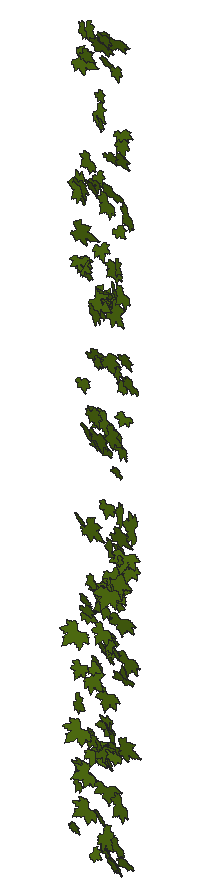
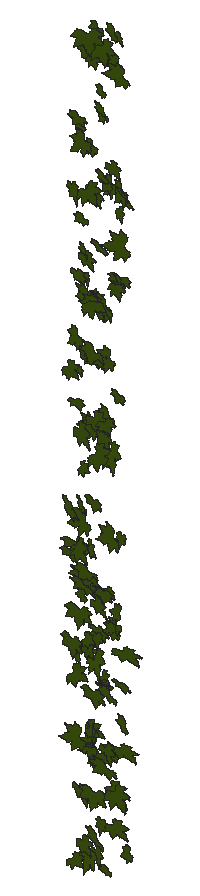
# SketchUp Ruby script. Lengths in inches.
U = 1.inch
M = Sketchup.active_model
def pt(a) = Geom::Point3d.new(a.map { |v| v * U })
def face(e, loops, mat)
  f = e.add_face(loops[0].map { |a| pt(a) })
  loops[1..].each { |l| e.add_face(l.map { |a| pt(a) }).erase! }
  f.material = f.back_material = mat if mat
  f
end
# faces: each face lists its corners as indices into pts; further lists are holes
def faces(e, pts, list, mat = nil) = list.each { |f| face(e, (f[0].is_a?(Array) ? f : [f]).map { |l| l.map { |i| pts[i] } }, mat) }
# xy, xz, yz: faces in a plane at the given z, y or x. An outline is a flat list of corners, or four numbers for a rectangle; further outlines are holes
def ring(l) = l.size == 4 ? [[l[0], l[1]], [l[2], l[1]], [l[2], l[3]], [l[0], l[3]]] : l.each_slice(2).to_a
def flat(e, list, mat, &to3) = list.each { |f| face(e, (f[0].is_a?(Array) ? f : [f]).map { |l| ring(l).map { |u, v| to3.(u, v) } }, mat) }
def xy(e, z, list, mat = nil) = flat(e, list, mat) { |x, y| [x, y, z] }
def xz(e, y, list, mat = nil) = flat(e, list, mat) { |x, z| [x, y, z] }
def yz(e, x, list, mat = nil) = flat(e, list, mat) { |y, z| [x, y, z] }
def lines(e, pts, list) = list.each { |a, b| e.add_line(pt(pts[a]), pt(pts[b])) }
# prism: a flat outline (further loops are holes) pulled along v
def prism(e, loops, v, mat = nil)
  f = face(e, loops, mat); d = Geom::Vector3d.new(v.map { |x| x * U })
  f.pushpull(f.normal.samedirection?(d) ? d.length : -d.length)
end
def box(e, o, s, mat = nil) = prism(e, [[o, [o[0] + s[0], o[1], o[2]], [o[0] + s[0], o[1] + s[1], o[2]], [o[0], o[1] + s[1], o[2]]]], [0, 0, s[2]], mat)
def at(x, y, z, deg = 0) = Geom::Transformation.translation(pt([x, y, z])) * Geom::Transformation.rotation(ORIGIN, Z_AXIS, deg.degrees)
def axes(o, x, y, z) = Geom::Transformation.new([*x, 0, *y, 0, *z, 0, *pt(o).to_a, 1])
def part(name) = M.definitions.add(name)
# library, detail: a bought-in or finely detailed component or shape, given as its bounding box
def library(name, o, s) = part(name).tap { |d| box(d.entities, o, s) }
def detail(e, o, s) = box(e.add_group.entities, o, s)
def put(e, d, t, mat = nil) = e.add_instance(d, t).tap { |i| i.material = mat if mat }
def group(e, t, mat = nil) = e.add_group.tap { |g| g.transformation = t; g.material = mat if mat }.entities
root = M.entities
M.materials.add("[Vegetation Blur 03]").color = [83, 114, 18]
c1 = part("ivy")
xy(c1.entities,0,[[0.782,0,0.786,0,0.787,0.005,0.789,0.009,0.821,0.072,0.875,0.147,1.001,0.272,1.073,0.331,1.137,0.363,1.178,0.379,1.223,0.384,1.272,0.383,1.311,0.374,1.36,0.355,1.399,0.334,1.491,0.285,1.541,0.244,1.583,0.199,1.617,0.15,1.64,0.128,1.662,0.115,1.717,0.105,1.745,0.093,1.784,0.054,1.819,0.057,1.854,0.064,1.882,0.075,1.896,0.074,1.91,0.071,1.937,0.063,1.964,0.053,1.99,0.038,2.016,0.015,2.034,0.002,2.04,0,2.038,0.003,2.036,0.007,2.033,0.038,2.036,0.068,2.045,0.1,2.055,0.116,2.064,0.123,2.077,0.129,2.088,0.129,2.106,0.132,2.118,0.13,2.179,0.132,2.207,0.133,2.225,0.133,2.242,0.138,2.22,0.162,2.207,0.186,2.206,0.213,2.212,0.236,2.228,0.262,2.247,0.274,2.298,0.283,2.355,0.294,2.37,0.296,2.376,0.295,2.377,0.3,2.377,0.303,2.385,0.329,2.411,0.37,2.426,0.392,2.449,0.407,2.511,0.426,2.561,0.444,2.619,0.466,2.589,0.469,2.561,0.476,2.501,0.5,2.449,0.516,2.424,0.523,2.401,0.535,2.377,0.556,2.372,0.568,2.36,0.575,2.268,0.586,2.225,0.592,2.207,0.599,2.194,0.61,2.143,0.65,2.13,0.664,2.122,0.682,2.123,0.7,2.13,0.719,2.148,0.75,2.17,0.781,2.195,0.807,2.221,0.828,2.284,0.874,2.291,0.88,2.288,0.887,2.276,0.9,2.267,0.916,2.265,0.933,2.273,0.967,2.292,1.002,2.313,1.03,2.334,1.054,2.348,1.067,2.358,1.074,2.363,1.076,2.362,1.081,2.35,1.094,2.347,1.11,2.35,1.143,2.359,1.18,2.385,1.254,2.415,1.324,2.448,1.393,2.45,1.4,2.446,1.398,2.44,1.394,2.427,1.383,2.402,1.36,2.376,1.339,2.345,1.324,2.305,1.309,2.282,1.303,2.273,1.306,2.245,1.294,2.212,1.287,2.187,1.291,2.163,1.301,2.142,1.316,2.134,1.327,2.124,1.325,2.09,1.292,2.053,1.259,2.014,1.234,1.973,1.215,1.954,1.21,1.931,1.208,1.909,1.212,1.893,1.22,1.879,1.233,1.872,1.248,1.867,1.281,1.864,1.319,1.821,1.258,1.773,1.197,1.726,1.141,1.698,1.121,1.679,1.116,1.666,1.117,1.647,1.122,1.632,1.129,1.62,1.141,1.617,1.154,1.617,1.219,1.621,1.254,1.623,1.268,1.623,1.281,1.618,1.314,1.606,1.346,1.603,1.375,1.607,1.403,1.603,1.467,1.599,1.499,1.605,1.525,1.614,1.552,1.629,1.577,1.635,1.589,1.629,1.587,1.618,1.582,1.596,1.566,1.581,1.556,1.568,1.552,1.557,1.55,1.545,1.553,1.531,1.562,1.522,1.572,1.504,1.591,1.486,1.611,1.474,1.631,1.457,1.666,1.455,1.684,1.457,1.698,1.452,1.715,1.444,1.728,1.424,1.754,1.419,1.772,1.423,1.786,1.434,1.819,1.444,1.848,1.446,1.855,1.44,1.861,1.43,1.867,1.386,1.904,1.349,1.948,1.326,1.973,1.31,1.995,1.288,2.048,1.284,2.153,1.287,2.254,1.284,2.255,1.282,2.253,1.278,2.247,1.274,2.237,1.266,2.216,1.226,2.125,1.208,2.076,1.184,2.033,1.155,1.984,1.135,1.942,1.111,1.899,1.083,1.861,1.053,1.85,1.059,1.83,1.061,1.809,1.056,1.79,1.049,1.767,1.04,1.749,1.018,1.733,0.994,1.726,0.942,1.734,0.95,1.6875,0.944,1.645,0.932,1.608,0.911,1.585,0.881,1.58,0.854,1.582,0.828,1.588,0.785,1.618,0.773,1.625,0.775,1.614,0.779,1.598,0.796,1.502,0.818,1.402,0.861,1.283,0.882,1.224,0.894,1.174,0.892,1.148,0.886,1.123,0.881,1.107,0.872,1.099,0.849,1.094,0.818,1.092,0.789,1.098,0.762,1.107,0.753,1.113,0.721,1.139,0.698,1.163,0.678,1.194,0.665,1.224,0.628,1.28,0.612,1.312,0.606,1.327,0.606,1.314,0.599,1.282,0.594,1.267,0.581,1.256,0.544,1.245,0.512,1.244,0.473,1.249,0.444,1.256,0.382,1.288,0.339,1.306,0.324,1.316,0.317,1.324,0.309,1.326,0.27,1.314,0.227,1.313,0.185,1.3125,0.152,1.317,0.122,1.328,0.092,1.345,0.073,1.353,0.079,1.338,0.092,1.308,0.117,1.249,0.13,1.215,0.139,1.164,0.147,1.148,0.157,1.136,0.163,1.122,0.174,1.086,0.177,1.067,0.182,1.054,0.186,1.043,0.191,1.038,0.211,1.028,0.237,1.005,0.25,0.974,0.253,0.96,0.25,0.944,0.242,0.914,0.243,0.906,0.249,0.902,0.26,0.894,0.289,0.88,0.307,0.873,0.322,0.862,0.364,0.799,0.403,0.738,0.431,0.709,0.439,0.691,0.441,0.678,0.4375,0.66,0.428,0.645,0.394,0.623,0.303,0.594,0.255,0.581,0.214,0.577,0.179,0.573,0.173,0.568,0.175,0.561,0.167,0.55,0.141,0.523,0.113,0.503,0.077,0.49,0.045,0.486,0.026,0.485,0.019,0.486,0.011,0.483,0,0.471,0.014,0.467,0.044,0.455,0.058,0.447,0.07,0.438,0.097,0.411,0.125,0.394,0.158,0.377,0.174,0.366,0.182,0.359,0.185,0.361,0.242,0.331,0.253,0.316,0.258,0.303,0.262,0.283,0.274,0.278,0.308,0.274,0.341,0.252,0.366,0.226,0.366,0.222,0.37,0.22,0.38,0.221,0.395,0.221,0.425,0.216,0.45,0.207,0.465,0.192,0.473,0.178,0.484,0.15,0.489,0.116,0.483,0.089,0.468,0.058,0.45,0.035,0.435,0.018,0.429,0.011,0.434,0.012,0.438,0.014,0.469,0.019,0.542,0.016,0.581,0.015,0.612,0.027,0.68,0.055,0.696,0.057,0.712,0.052,0.73,0.045,0.741,0.036,0.766,0.014]])
put(root,c1,axes([122.65,173.7,114.2],[0.52837,-0.04737,-0.26503],[-0.32337,-0.22367,-0.42312],[0.03764,-1.25647,0.08531]),"[Vegetation Blur 03]")
put(root,c1,axes([123.47,173.7,137.38],[0.14321,-0.30149,-0.44399],[-0.54717,0.20081,-0.13901],[-0.13425,-1.14006,0.09293]),"[Vegetation Blur 03]")
put(root,c1,axes([122.48,173.7,103.37],[0.20518,-0.11933,0.20995],[0.26085,-0.0065,-0.17038],[-0.03866,-0.67709,-0.03537]),"[Vegetation Blur 03]")
put(root,c1,axes([122.83,173.7,109.21],[0.5099,-0.05447,-0.26558],[-0.32487,-0.20771,-0.40876],[0.03235,-1.22728,0.08097]),"[Vegetation Blur 03]")
put(root,c1,axes([123.1,173.7,136.44],[0.23798,-0.09799,-0.20106],[-0.2294,0.19812,-0.19604],[-0.10166,-0.67644,-0.02829]),"[Vegetation Blur 03]")
put(root,c1,axes([123.13,173.7,107.16],[0.44315,0.00145,-0.39097],[-0.47521,0.17095,-0.35867],[-0.06051,-1.33197,-0.04646]),"[Vegetation Blur 03]")
put(root,c1,axes([122.87,173.7,119.7],[0.31001,-0.14403,-0.03677],[-0.03088,0.13304,-0.25536],[-0.0773,-0.63077,-0.04546]),"[Vegetation Blur 03]")
put(root,c1,axes([123.07,173.7,132.65],[0.35037,-0.01321,-0.20166],[-0.24181,0.16441,-0.28153],[-0.0512,-0.86678,-0.05033]),"[Vegetation Blur 03]")
put(root,c1,axes([122.59,173.7,132.83],[0.4392,0.07424,0.06802],[0.08567,-0.05755,-0.35857],[0.03015,-0.91812,0.02798]),"[Vegetation Blur 03]")
put(root,c1,axes([122.9375,173.7,106.1],[0.29646,-0.18293,-0.03481],[-0.04858,-0.02904,-0.25162],[-0.08579,-0.61566,0.02221]),"[Vegetation Blur 03]")
put(root,c1,axes([122.78,173.7,109.59],[0.06873,0.01711,0.34805],[0.41669,-0.19262,-0.05332],[-0.09114,-0.86777,0.0187]),"[Vegetation Blur 03]")
put(root,c1,axes([122.87,173.7,112.16],[0.41492,-0.08686,-0.03354],[-0.04844,-0.1605,-0.33372],[-0.03354,-0.84286,0.067]),"[Vegetation Blur 03]")
put(root,c1,axes([123.35,173.7,145.22],[0.22954,-0.17233,-0.19599],[-0.23774,0.09106,-0.19805],[-0.09034,-0.67751,0.02323]),"[Vegetation Blur 03]")
put(root,c1,axes([123.375,173.7,105.28],[0.4097,-0.04709,-0.34938],[-0.42867,-0.05903,-0.33358],[0.00494,-1.21793,0.02968]),"[Vegetation Blur 03]")
put(root,c1,axes([123.34,173.7,124.47],[0.46716,-0.062,-0.38996],[-0.44887,0.42109,-0.3687],[-0.16652,-1.30905,-0.10013]),"[Vegetation Blur 03]")
put(root,c1,axes([122.61,173.7,142.5],[0.13182,0.09274,0.49871],[0.61259,0.00582,-0.10802],[0.01227,-1.28635,0.03547]),"[Vegetation Blur 03]")
put(root,c1,axes([122.9,173.7,132.14],[0.09631,0.08819,0.32844],[0.40359,-0.08421,-0.07527],[-0.03009,-0.84734,0.04167]),"[Vegetation Blur 03]")
put(root,c1,axes([123.58,173.7,107.16],[0.31711,-0.08877,-0.37028],[-0.45541,-0.10498,-0.25583],[0.01733,-1.13422,0.05266]),"[Vegetation Blur 03]")
put(root,c1,axes([122.91,173.7,126.63],[0.33984,-0.05336,0.11192],[0.13528,-0.05673,-0.27786],[-0.03432,-0.75199,0.01302]),"[Vegetation Blur 03]")
put(root,c1,axes([122.62,173.7,133.74],[0.17934,-0.09894,0.51265],[0.6295,0.08025,-0.14425],[0.02442,-1.34184,-0.04643]),"[Vegetation Blur 03]")
put(root,c1,axes([122.7,173.7,136.88],[0.47833,-0.24749,0.17674],[0.22101,-0.01127,-0.40089],[-0.11188,-1.08043,-0.0363]),"[Vegetation Blur 03]")
put(root,c1,axes([123.54,173.7,138.62],[0.34594,-0.11487,-0.25725],[-0.31497,0.04827,-0.28551],[-0.05712,-0.96184,0.01639]),"[Vegetation Blur 03]")
put(root,c1,axes([123.07,173.7,114.89],[0.3213,-0.06644,0.14929],[0.18483,0.03966,-0.26218],[-0.01845,-0.75978,-0.02674]),"[Vegetation Blur 03]")
put(root,c1,axes([123.07,173.7,143.24],[0.18668,-0.06069,0.28857],[0.35478,0.02187,-0.15215],[-0.00434,-0.8225,-0.02534]),"[Vegetation Blur 03]")
put(root,c1,axes([123.27,173.7,115.22],[0.06463,-0.12992,0.26421],[0.32679,-0.06667,-0.0584],[-0.04465,-0.67604,-0.04502]),"[Vegetation Blur 03]")
put(root,c1,axes([123.14,173.7,114.36],[0.19136,0.01715,0.31471],[0.38568,-0.01715,-0.15606],[-0.00376,-0.88569,0.00911]),"[Vegetation Blur 03]")
put(root,c1,axes([123.7,173.7,125.49],[0.29858,0.09929,-0.17499],[-0.21887,0.06675,-0.24279],[0.01995,-0.75348,-0.04457]),"[Vegetation Blur 03]")
put(root,c1,axes([123.84,173.7,116.86],[0.2154,-0.10325,-0.19292],[-0.23671,0.04089,-0.17948],[-0.04859,-0.65681,0.01915]),"[Vegetation Blur 03]")
put(root,c1,axes([124.08,173.7,112.61],[0.12889,0.05373,-0.25764],[-0.31029,0.16238,-0.09807],[-0.06367,-0.68262,-0.04361]),"[Vegetation Blur 03]")
put(root,c1,axes([123.71,173.7,108.93],[0.42245,-0.13873,-0.23601],[-0.28027,0.15555,-0.34853],[-0.09809,-1.04193,-0.02061]),"[Vegetation Blur 03]")
put(root,c1,axes([123.35,173.7,144.58],[0.1212,0.00874,0.32904],[0.39357,-0.19062,-0.09576],[-0.08752,-0.84508,0.025]),"[Vegetation Blur 03]")
put(root,c1,axes([123.56,173.7,111.65],[0.07011,0.12287,0.23012],[0.28735,0.0166,-0.05971],[0.0224,-0.59768,0.04565]),"[Vegetation Blur 03]")
put(root,c1,axes([123.27,173.7,108.1],[0.22931,-0.05412,0.29769],[0.36487,-0.02596,-0.18795],[-0.02469,-0.88622,-0.01267]),"[Vegetation Blur 03]")
put(root,c1,axes([124.39,173.7,124.09],[0.19085,0.16255,-0.44019],[-0.54494,0.0863,-0.15236],[-0.01363,-1.17416,-0.07214]),"[Vegetation Blur 03]")
put(root,c1,axes([123.71,173.7,144.74],[0.51903,0.05216,-0.26245],[-0.32095,0.20906,-0.41624],[-0.03231,-1.23893,-0.08129]),"[Vegetation Blur 03]")
put(root,c1,axes([123.67,173.7,102.15],[0.08845,0.08211,0.23234],[0.28731,-0.04554,-0.07032],[-0.00952,-0.61175,0.03642]),"[Vegetation Blur 03]")
put(root,c1,axes([123.4,173.7,137.0625],[0.39765,-0.2594,0.13842],[0.18466,0.06494,-0.33421],[-0.10274,-0.88724,-0.06493]),"[Vegetation Blur 03]")
put(root,c1,axes([123.11,173.7,118.82],[0.30964,-0.0676,0.45983],[0.56279,-0.06237,-0.25387],[-0.0424,-1.3215,-0.01154]),"[Vegetation Blur 03]")
put(root,c1,axes([123.28,173.7,110.93],[0.19869,0.16598,0.44202],[0.5434,-0.20587,-0.15053],[-0.06748,-1.16914,0.08926]),"[Vegetation Blur 03]")
put(root,c1,axes([123.625,173.7,137.17],[0.34101,-0.13421,0.11002],[0.1371,0.00224,-0.28262],[-0.06025,-0.75456,-0.02041]),"[Vegetation Blur 03]")
put(root,c1,axes([123.26,173.7,107.34],[0.3778,0.16016,0.36511],[0.45377,-0.08873,-0.30663],[0.01685,-1.20168,0.0713]),"[Vegetation Blur 03]")
put(root,c1,axes([124.4375,173.7,131.13],[0.17466,-0.11177,-0.29584],[-0.34642,0.21964,-0.14928],[-0.11976,-0.79834,0.00035]),"[Vegetation Blur 03]")
put(root,c1,axes([123.45,173.7,128],[0.29936,-0.14494,0.31849],[0.3965,0.0953,-0.24142],[-0.00556,-1.00761,-0.06865]),"[Vegetation Blur 03]")
put(root,c1,axes([124.23,173.7,113.64],[0.40831,-0.04926,-0.36189],[-0.41615,0.39004,-0.3211],[-0.15494,-1.17746,-0.09123]),"[Vegetation Blur 03]")
put(root,c1,axes([123.72,173.7,116.53],[0.44619,-0.06474,-0.00167],[-0.00306,-0.02944,-0.36486],[-0.03138,-0.91771,0.01182]),"[Vegetation Blur 03]")
put(root,c1,axes([123.44,173.7,125.14],[0.40671,-0.14437,0.24599],[0.29835,-0.08915,-0.33679],[-0.0822,-1.03788,-0.00529]),"[Vegetation Blur 03]")
put(root,c1,axes([123.68,173.7,130.79],[0.45964,-0.254,0.03008],[0.03689,-0.00973,-0.3884],[-0.12342,-0.94883,-0.00407]),"[Vegetation Blur 03]")
put(root,c1,axes([124.86,173.7,131.72],[0.10531,0.2061,-0.4524],[-0.56328,0.04564,-0.08406],[-0.00345,-1.16018,-0.08367]),"[Vegetation Blur 03]")
put(root,c1,axes([124.03,173.7,104.83],[0.35108,-0.18402,-0.07774],[-0.07773,0.15757,-0.29247],[-0.10502,-0.7318,-0.04343]),"[Vegetation Blur 03]")
put(root,c1,axes([124.41,173.7,125.68],[0.41789,-0.06408,-0.38347],[-0.47,0.02266,-0.34176],[-0.02893,-1.29377,0.01301]),"[Vegetation Blur 03]")
put(root,c1,axes([123.96,173.7,127.7],[0.0683,-0.05119,0.27634],[0.33407,-0.11649,-0.05839],[-0.06049,-0.70118,-0.01047]),"[Vegetation Blur 03]")
put(root,c1,axes([123.85,173.7,137.29],[0.21707,0.00977,0.22202],[0.26718,-0.14285,-0.17301],[-0.05136,-0.70178,0.03831]),"[Vegetation Blur 03]")
put(root,c1,axes([123.5625,173.7,130.47],[0.16468,0.13945,0.51477],[0.63081,-0.17776,-0.12684],[-0.06707,-1.32961,0.07095]),"[Vegetation Blur 03]")
put(root,c1,axes([123.84,173.7,140.37],[0.13518,0.07282,0.36034],[0.43243,-0.22734,-0.10083],[-0.09589,-0.9226,0.05329]),"[Vegetation Blur 03]")
put(root,c1,axes([124,173.7,141.61],[0.18338,-0.0476,0.19783],[0.23906,-0.08339,-0.15076],[-0.04624,-0.61987,0.00509]),"[Vegetation Blur 03]")
put(root,c1,axes([124.49,173.7,116.17],[0.36665,-0.19895,-0.32997],[-0.4044,0.08632,-0.30749],[-0.09631,-1.11984,0.03492]),"[Vegetation Blur 03]")
put(root,c1,axes([124.36,173.7,103.47],[0.35757,-0.14861,-0.22341],[-0.2596,0.18993,-0.29662],[-0.11295,-0.907,-0.02551]),"[Vegetation Blur 03]")
put(root,c1,axes([124.26,173.7,114.33],[0.32932,-0.07979,-0.11263],[-0.13041,0.12861,-0.26832],[-0.05951,-0.72344,-0.03528]),"[Vegetation Blur 03]")
put(root,c1,axes([123.625,173.7,124.36],[0.58972,-0.25941,0.10506],[0.13617,0.04808,-0.49046],[-0.11798,-1.24117,-0.04096]),"[Vegetation Blur 03]")
put(root,c1,axes([124.47,173.7,143.77],[0.26625,0.02526,-0.1848],[-0.22371,0.14694,-0.21152],[-0.03714,-0.70407,-0.05077]),"[Vegetation Blur 03]")
put(root,c1,axes([124.95,173.7,109.84],[0.13243,-0.0083,-0.40164],[-0.49158,0.04791,-0.10811],[-0.02353,-1.04762,-0.00176]),"[Vegetation Blur 03]")
put(root,c1,axes([124.04,173.7,140.57],[0.32682,-0.209,0.08086],[0.0994,-0.02803,-0.27901],[-0.10124,-0.70219,-0.01293]),"[Vegetation Blur 03]")
put(root,c1,axes([123.89,173.7,133.73],[0.33502,0.02499,0.20079],[0.2423,-0.1873,-0.26561],[-0.04435,-0.83458,0.06562]),"[Vegetation Blur 03]")
put(root,c1,axes([124.86,173.7,131.3125],[0.07838,0.01913,-0.25028],[-0.30675,-0.00782,-0.06408],[0.00599,-0.6513,-0.00658]),"[Vegetation Blur 03]")
put(root,c1,axes([124.68,173.7,137.28],[0.33022,0.14446,-0.3444],[-0.42741,0.15711,-0.26261],[-0.01782,-1.09139,-0.08339]),"[Vegetation Blur 03]")
put(root,c1,axes([124.17,173.7,114.61],[0.48596,-0.138,-0.11802],[-0.15256,-0.12597,-0.39525],[-0.04619,-1.03571,0.0638]),"[Vegetation Blur 03]")
put(root,c1,axes([124.32,173.7,131.2],[0.33133,0.03179,-0.00697],[-0.01113,0.11989,-0.26643],[0.0137,-0.67142,-0.0479]),"[Vegetation Blur 03]")
put(root,c1,axes([125,173.7,118.95],[0.13696,-0.09293,-0.32969],[-0.38837,0.22901,-0.11762],[-0.11998,-0.84735,0.00437]),"[Vegetation Blur 03]")
put(root,c1,axes([124.53,173.7,109.54],[0.33215,-0.12492,-0.16924],[-0.19211,0.18741,-0.2729],[-0.09889,-0.78367,-0.03828]),"[Vegetation Blur 03]")
put(root,c1,axes([124.1,173.7,144.86],[0.38814,-0.14356,0.10109],[0.12917,0.04667,-0.31993],[-0.05936,-0.83711,-0.03517]),"[Vegetation Blur 03]")
put(root,c1,axes([123.92,173.7,106.25],[0.6157,0.01002,0.02515],[0.03061,0.04996,-0.50212],[0.00607,-1.26758,-0.01959]),"[Vegetation Blur 03]")
put(root,c1,axes([123.77,173.7,108.03],[0.55674,-0.05035,0.19483],[0.23814,-0.03752,-0.45478],[-0.02967,-1.24598,0.00582]),"[Vegetation Blur 03]")
put(root,c1,axes([124.26,173.7,145.05],[0.59461,0.12109,-0.18026],[-0.22736,0.18289,-0.48022],[0.02354,-1.29241,-0.08484]),"[Vegetation Blur 03]")
put(root,c1,axes([124.11,173.7,130.58],[0.10294,0.13872,0.40661],[0.50198,0.02961,-0.08624],[0.02785,-1.04645,0.05146]),"[Vegetation Blur 03]")
put(root,c1,axes([124.48,173.7,136.94],[0.49987,-0.22483,-0.22694],[-0.27931,0.04426,-0.41667],[-0.10606,-1.17624,0.0277]),"[Vegetation Blur 03]")
put(root,c1,axes([125.13,173.7,113.54],[0.04662,-0.02211,-0.24119],[-0.29524,-0.03871,-0.03745],[0.01692,-0.61444,0.01104]),"[Vegetation Blur 03]")
put(root,c1,axes([125.04,173.7,113.9],[0.21141,-0.03642,-0.34067],[-0.40654,0.204,-0.17147],[-0.09632,-0.94099,-0.02399]),"[Vegetation Blur 03]")
put(root,c1,axes([125.14,173.7,114.15],[0.07372,0.06524,-0.26494],[-0.3259,0.04312,-0.05873],[-0.01352,-0.68368,-0.02899]),"[Vegetation Blur 03]")
put(root,c1,axes([124.84,173.7,109.72],[0.32192,-0.21102,-0.29136],[-0.33943,0.22769,-0.27574],[-0.15085,-0.96265,-0.00135]),"[Vegetation Blur 03]")
put(root,c1,axes([124.2,173.7,111.29],[0.58789,-0.11281,-0.04556],[-0.05859,-0.05769,-0.48112],[-0.05185,-1.21383,0.0271]),"[Vegetation Blur 03]")
put(root,c1,axes([124.33,173.7,120.92],[0.43658,-0.10423,0.00392],[0.00224,-0.04583,-0.35826],[-0.05083,-0.89729,0.01784]),"[Vegetation Blur 03]")
put(root,c1,axes([124.26,173.7,116.72],[0.62885,-0.10059,-0.07918],[-0.103,-0.17922,-0.50906],[-0.03454,-1.29703,0.07648]),"[Vegetation Blur 03]")
put(root,c1,axes([124.09,173.7,103.21],[0.24806,0.03915,0.43187],[0.51673,-0.28046,-0.19369],[-0.11561,-1.16947,0.06091]),"[Vegetation Blur 03]")
put(root,c1,axes([124.89,173.7,116.78],[0.30881,-0.07275,-0.21101],[-0.25864,0.02403,-0.25343],[-0.03462,-0.82843,0.01118]),"[Vegetation Blur 03]")
put(root,c1,axes([124.42,173.7,138.69],[0.29342,-0.08692,0.17033],[0.21238,0.06683,-0.23833],[-0.01533,-0.73794,-0.04165]),"[Vegetation Blur 03]")
put(root,c1,axes([124.03,173.7,128.21],[0.52256,-0.08904,0.24501],[0.30058,-0.01277,-0.42774],[-0.04062,-1.24009,-0.01319]),"[Vegetation Blur 03]")
put(root,c1,axes([124.53,173.7,107.625],[0.27556,-0.19726,0.13683],[0.17351,-0.01114,-0.23526],[-0.08482,-0.66366,-0.03672]),"[Vegetation Blur 03]")
put(root,c1,axes([124.5,173.7,113.52],[0.23663,-0.00308,0.21961],[0.25991,-0.18831,-0.18695],[-0.06967,-0.71292,0.04843]),"[Vegetation Blur 03]")
put(root,c1,axes([125.38,173.7,122.76],[0.04516,0.08728,-0.24004],[-0.29622,0.06188,-0.03358],[-0.02362,-0.6092,-0.0378]),"[Vegetation Blur 03]")
put(root,c1,axes([124.97,173.7,133.52],[0.38178,-0.11889,-0.25625],[-0.31299,0.05919,-0.31491],[-0.06294,-1.01546,0.01165]),"[Vegetation Blur 03]")
put(root,c1,axes([125.13,173.7,103.86],[0.3336,-0.07994,-0.30777],[-0.37102,0.14358,-0.27372],[-0.07791,-1.02608,-0.01433]),"[Vegetation Blur 03]")
put(root,c1,axes([125.05,173.7,132.32],[0.23472,-0.16453,-0.13977],[-0.15775,0.13898,-0.20218],[-0.10411,-0.58153,-0.00877]),"[Vegetation Blur 03]")
put(root,c1,axes([125.09,173.7,108.46],[0.296,-0.08214,-0.20649],[-0.25613,-0.08908,-0.23898],[-0.00188,-0.79632,0.04803]),"[Vegetation Blur 03]")
put(root,c1,axes([124.64,173.7,102.66],[0.4103,-0.202,-0.00421],[0.00893,0.12198,-0.34084],[-0.09789,-0.83552,-0.04874]),"[Vegetation Blur 03]")
put(root,c1,axes([124.49,173.7,103.04],[0.61856,-0.3329,-0.06965],[-0.05285,0.26763,-0.51381],[-0.1751,-1.25675,-0.09097]),"[Vegetation Blur 03]")
put(root,c1,axes([124.36,173.7,117.02],[0.386,0.08915,0.27036],[0.33331,-0.03157,-0.31533],[0.02283,-1.04625,0.03255]),"[Vegetation Blur 03]")
put(root,c1,axes([124.46,173.7,108.09],[0.30498,-0.11066,0.28031],[0.34736,0.05892,-0.24807],[-0.01408,-0.94337,-0.04838]),"[Vegetation Blur 03]")
put(root,c1,axes([125.375,173.7,124.82],[0.38094,-0.16652,-0.42659],[-0.51102,0.22607,-0.31784],[-0.13644,-1.3116,-0.00062]),"[Vegetation Blur 03]")
put(root,c1,axes([125.51,173.7,118.9375],[0.2944,-0.05147,-0.44172],[-0.52796,0.2576,-0.2391],[-0.12176,-1.24142,-0.0313]),"[Vegetation Blur 03]")
put(root,c1,axes([125.69,173.7,120.95],[0.09708,-0.16375,-0.35064],[-0.41312,0.26056,-0.09533],[-0.14231,-0.86813,0.03753]),"[Vegetation Blur 03]")
put(root,c1,axes([124.49,173.7,123.99],[0.19561,-0.07372,0.44835],[0.54629,-0.12238,-0.16192],[-0.06809,-1.19373,-0.01109]),"[Vegetation Blur 03]")
put(root,c1,axes([125.72,173.7,112.41],[0.11047,0.20453,-0.35161],[-0.44126,-0.0065,-0.09294],[0.02783,-0.9152,-0.07792]),"[Vegetation Blur 03]")
put(root,c1,axes([124.3,173.7,116.8125],[0.58138,0.04851,0.24502],[0.30111,-0.07156,-0.47365],[0.00495,-1.34457,0.03405]),"[Vegetation Blur 03]")
put(root,c1,axes([124.89,173.7,143.36],[0.32177,-0.10077,0.13804],[0.16444,-0.08743,-0.26534],[-0.06299,-0.74292,0.0125]),"[Vegetation Blur 03]")
put(root,c1,axes([124.95,173.7,134.86],[0.2013,0.04338,0.20783],[0.25534,-0.0094,-0.16443],[0.00948,-0.6679,0.01581]),"[Vegetation Blur 03]")
put(root,c1,axes([125.01,173.7,118.22],[0.28684,-0.06236,0.1063],[0.12625,-0.08285,-0.23456],[-0.04409,-0.64295,0.01992]),"[Vegetation Blur 03]")
put(root,c1,axes([124.66,173.7,116.17],[0.3314,0.11464,0.31783],[0.39311,-0.13672,-0.26526],[-0.0151,-1.04335,0.06968]),"[Vegetation Blur 03]")
put(root,c1,axes([125.1,173.7,115.56],[0.07858,-0.01385,0.24493],[0.29907,-0.05144,-0.06436],[-0.02588,-0.6363,-0.00013]),"[Vegetation Blur 03]")
put(root,c1,axes([125.67,173.7,102.8125],[0.1696,0.1381,-0.24942],[-0.31204,0.02191,-0.13942],[0.02307,-0.7189,-0.05216]),"[Vegetation Blur 03]")
put(root,c1,axes([125.0625,173.7,132.93],[0.07908,0.01608,0.29029],[0.3424,-0.20709,-0.06032],[-0.09663,-0.72064,0.02381]),"[Vegetation Blur 03]")
put(root,c1,axes([124.54,173.7,130.52],[0.31957,-0.02324,0.46113],[0.55443,-0.24575,-0.25788],[-0.10943,-1.31297,0.04011]),"[Vegetation Blur 03]")
put(root,c1,axes([124.82,173.7,115.3],[0.62015,-0.02976,-0.03519],[-0.04222,0.07375,-0.50547],[-0.01689,-1.27709,-0.02837]),"[Vegetation Blur 03]")
put(root,c1,axes([125.05,173.7,127.85],[0.25768,-0.12141,0.16925],[0.19637,-0.14245,-0.21521],[-0.08903,-0.66558,0.01519]),"[Vegetation Blur 03]")
put(root,c1,axes([124.72,173.7,138.72],[0.41952,-0.13561,0.24997],[0.31292,0.12999,-0.33871],[-0.01528,-1.06095,-0.07345]),"[Vegetation Blur 03]")
put(root,c1,axes([125.3,173.7,106.22],[0.52518,-0.29878,-0.23016],[-0.2856,0.04291,-0.44284],[-0.13799,-1.22592,0.0406]),"[Vegetation Blur 03]")
put(root,c1,axes([125.53,173.7,127.49],[0.2496,-0.10992,-0.13236],[-0.16418,0.00788,-0.20725],[-0.04691,-0.61248,0.02109]),"[Vegetation Blur 03]")
put(root,c1,axes([125.4,173.7,132.38],[0.42696,-0.16855,-0.18226],[-0.22665,-0.00186,-0.3534],[-0.07216,-0.99152,0.03164]),"[Vegetation Blur 03]")
put(root,c1,axes([125.42,173.7,125.82],[0.33208,0.00162,-0.09351],[-0.114,-0.06757,-0.26985],[0.01145,-0.71971,0.02513]),"[Vegetation Blur 03]")
put(root,c1,axes([125.05,173.7,140.02],[0.3458,0.03513,0.16386],[0.2014,-0.03386,-0.28195],[0.00648,-0.82214,0.01861]),"[Vegetation Blur 03]")
put(root,c1,axes([125.09,173.7,118.63],[0.56687,0.06013,-0.01984],[-0.01943,-0.18427,-0.45761],[0.03267,-1.15295,0.0721]),"[Vegetation Blur 03]")
put(root,c1,axes([125.99,173.7,127.74],[0.21346,0.05085,-0.33078],[-0.40485,0.09932,-0.17162],[-0.03132,-0.93739,-0.03613]),"[Vegetation Blur 03]")
put(root,c1,axes([124.84,173.7,119.1],[0.31154,-0.18802,0.42817],[0.53015,-0.00865,-0.25753],[-0.0503,-1.25557,-0.06234]),"[Vegetation Blur 03]")
put(root,c1,axes([125.16,173.7,139.62],[0.34903,-0.06561,0.18456],[0.21828,-0.15404,-0.28357],[-0.06714,-0.84183,0.0375]),"[Vegetation Blur 03]")
put(root,c1,axes([125.5,173.7,112.33],[0.10915,-0.09215,0.23401],[0.27778,-0.14927,-0.09555],[-0.08399,-0.61343,-0.0119]),"[Vegetation Blur 03]")
put(root,c1,axes([126.52,173.7,120.7],[0.10352,-0.20906,-0.49577],[-0.59692,0.27823,-0.10147],[-0.15173,-1.23717,0.06096]),"[Vegetation Blur 03]")
put(root,c1,axes([125.71,173.7,136.71],[0.46455,-0.28541,-0.24702],[-0.29064,0.17394,-0.39567],[-0.16241,-1.12761,0.00149]),"[Vegetation Blur 03]")
put(root,c1,axes([125.13,173.7,108.02],[0.20638,-0.06433,0.46905],[0.57546,0.04752,-0.16762],[0.01121,-1.25569,-0.03037]),"[Vegetation Blur 03]")
put(root,c1,axes([125.28,173.7,128.62],[0.36896,-0.184,0.21842],[0.27276,0.00042,-0.30684],[-0.07226,-0.93795,-0.04299]),"[Vegetation Blur 03]")
put(root,c1,axes([125.51,173.7,118.04],[0.4452,0.01529,-0.01974],[-0.02317,-0.10578,-0.36101],[0.01016,-0.91136,0.04157]),"[Vegetation Blur 03]")
put(root,c1,axes([125.41,173.7,113.57],[0.60359,-0.16861,-0.0634],[-0.07511,0.04962,-0.497],[-0.08431,-1.25133,-0.01117]),"[Vegetation Blur 03]")
